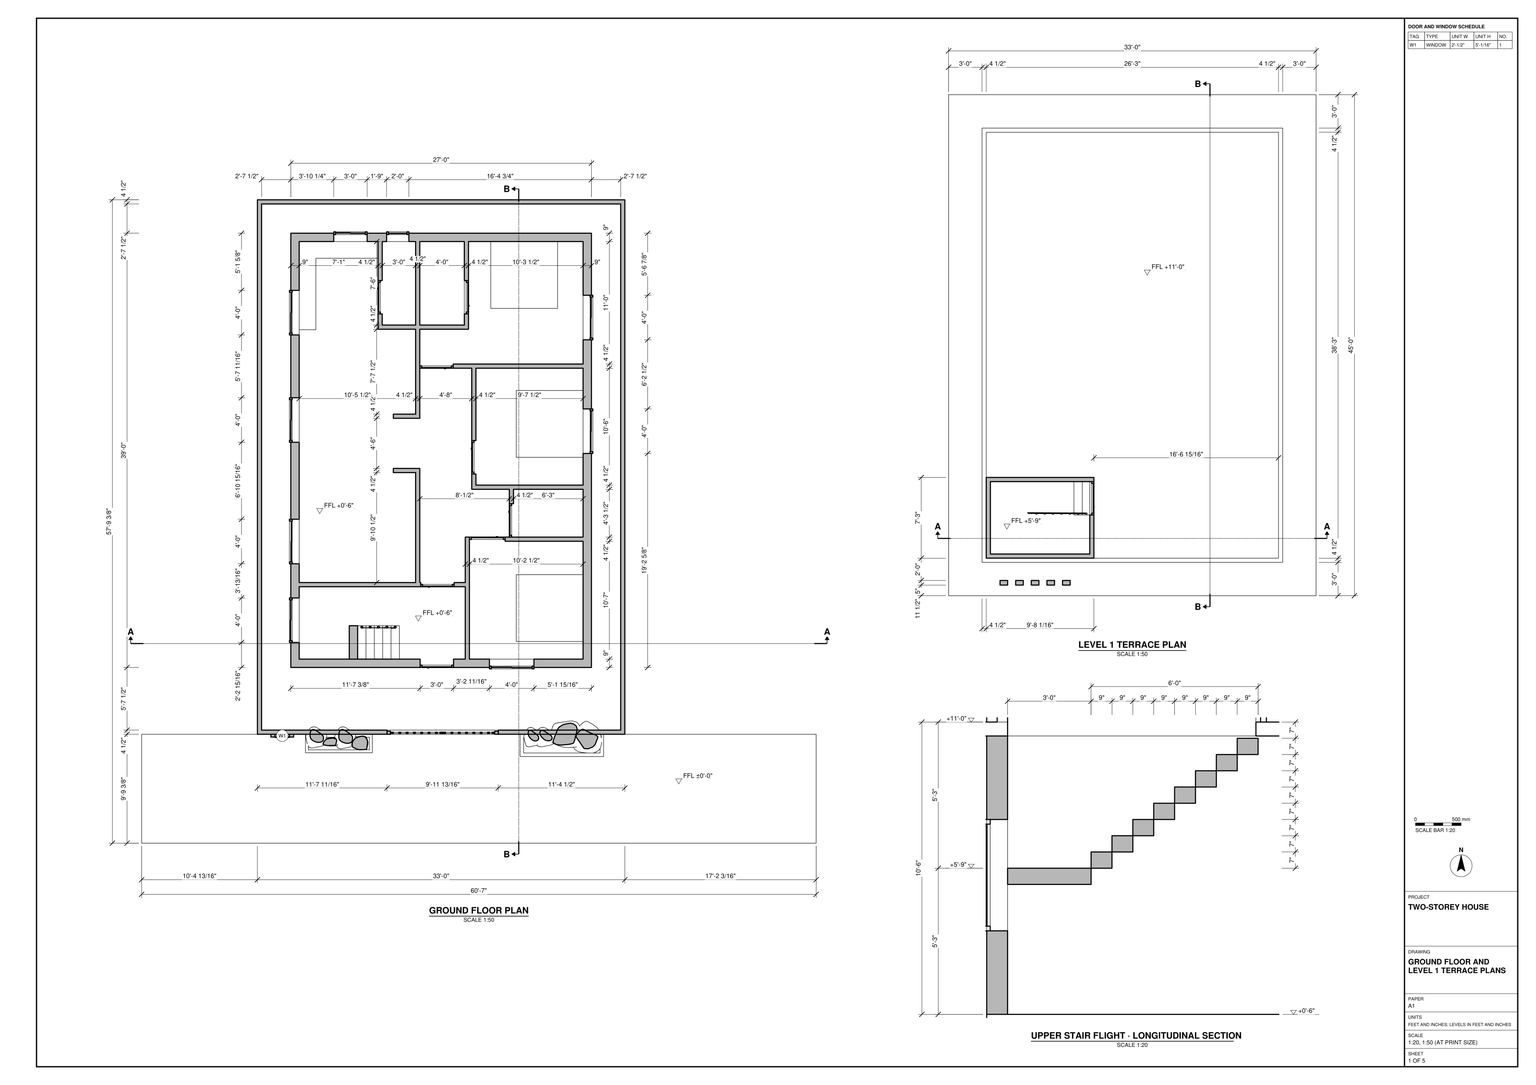
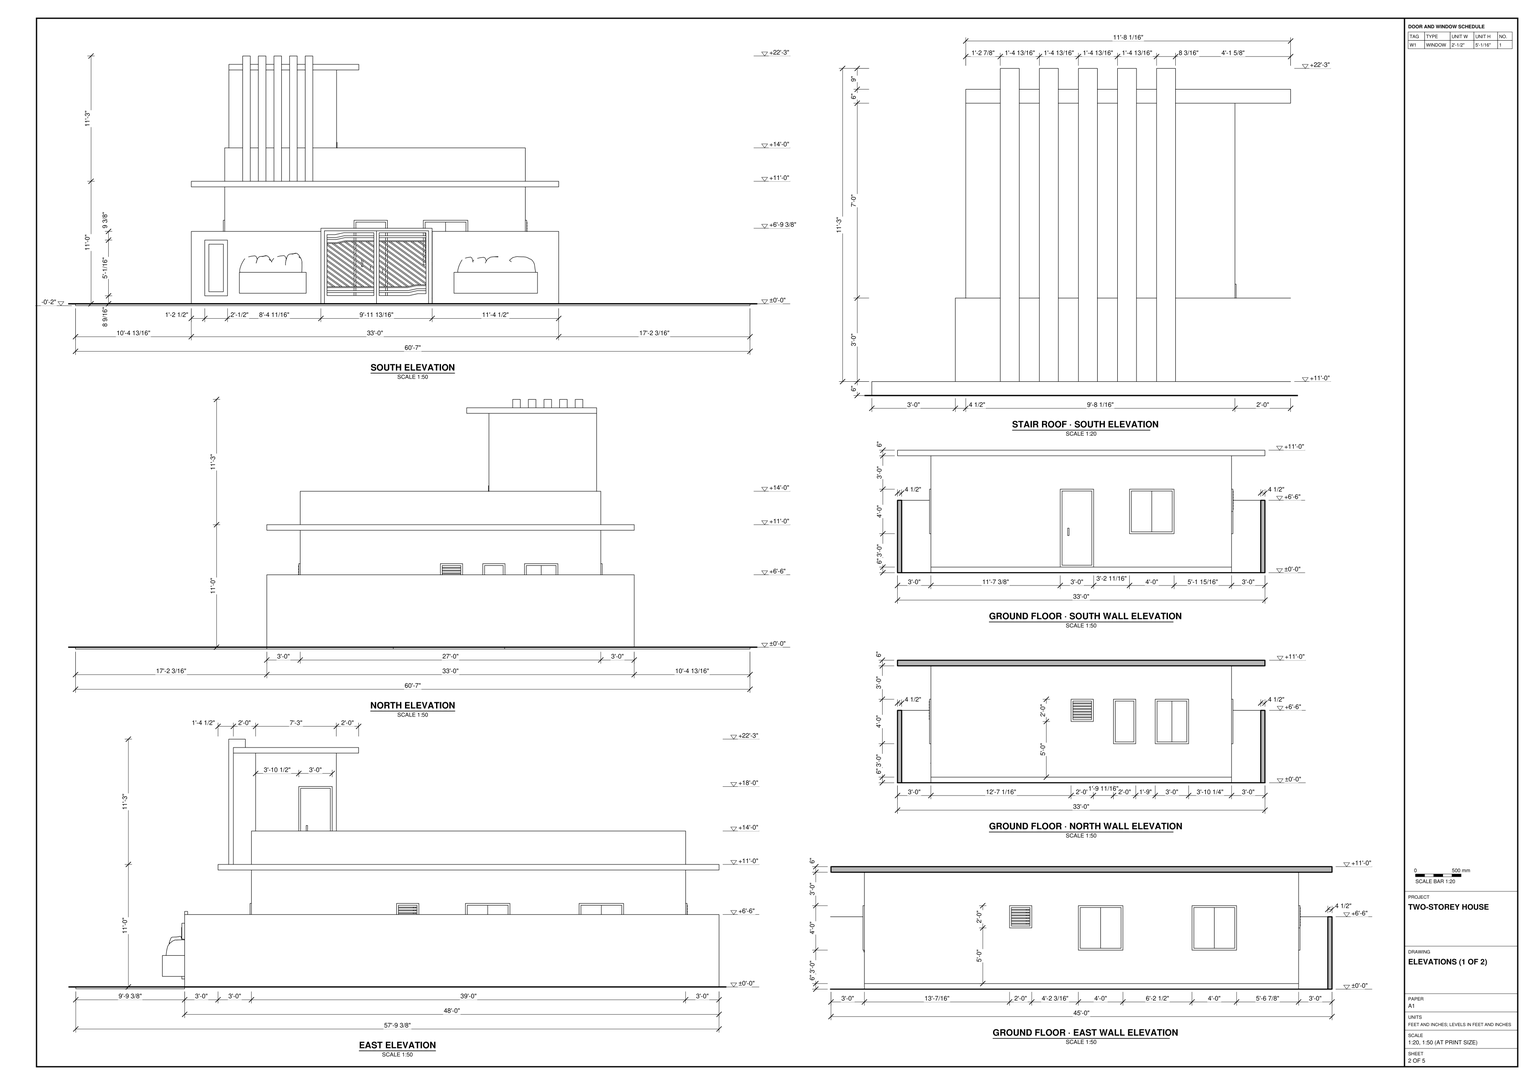
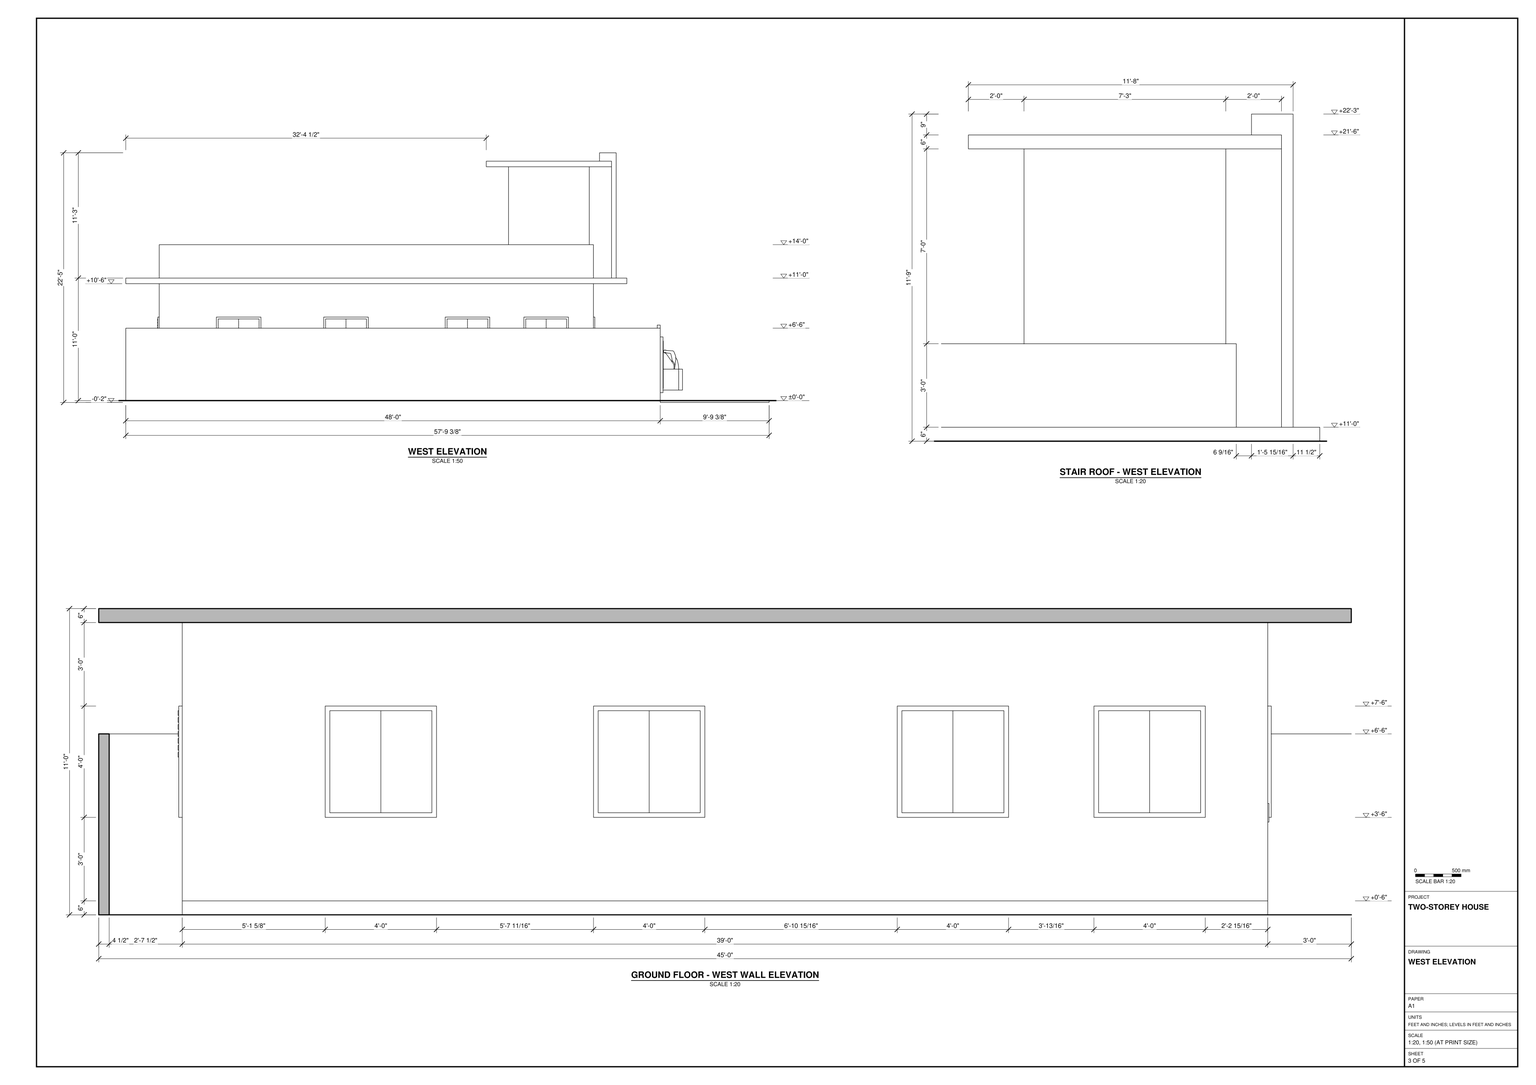
Build the house and its site in SketchUp using task_files/diagram_01.pdf. Work in feet and inches. The overall model, including the ground strip across the front, is 60'-7" wide, 57'-9 3/8" deep and 22'-5" high. Use ±0'-0" as the ground datum and +11'-0" as the terrace level. Set the interior floor at +0'-6", as shown in the ground-floor plan.

Lay out the 27'-0" by 39'-0" house footprint with 9" exterior walls and 4 1/2" interior partitions. Follow the plan for the rooms, connecting passages, built-in joinery and main furniture. Use the individual wall elevations to locate the entrance door, windows and vents. Model the floor slab and the stair near the south entrance, including the intermediate landing at +5'-9". Continue the stair to the enclosure at the southwest corner of the terrace. Show the projecting terrace slab, its inset parapet, and the enclosure’s flat roof and vertical fins.

Model the boundary walls and the double-leaf gate facing south, with a planted box on either side. Decor and loose items, including the plants, may be any suitable library components. Keep shell elements such as walls, slabs and roofs, and each furniture or joinery piece, in separate groups or components. Use components for repeated parts. Save one SketchUp model as output_files/two_storey_house_with_a_roof_terrace_and_gated_frontage.skp.

# SketchUp Ruby script. Lengths in inches.
U = 1.inch
M = Sketchup.active_model
def pt(a) = Geom::Point3d.new(a.map { |v| v * U })
def face(e, loops, mat)
  f = e.add_face(loops[0].map { |a| pt(a) })
  loops[1..].each { |l| e.add_face(l.map { |a| pt(a) }).erase! }
  f.material = f.back_material = mat if mat
  f
end
# faces: each face lists its corners as indices into pts; further lists are holes
def faces(e, pts, list, mat = nil) = list.each { |f| face(e, (f[0].is_a?(Array) ? f : [f]).map { |l| l.map { |i| pts[i] } }, mat) }
# xy, xz, yz: faces in a plane at the given z, y or x. An outline is a flat list of corners, or four numbers for a rectangle; further outlines are holes
def ring(l) = l.size == 4 ? [[l[0], l[1]], [l[2], l[1]], [l[2], l[3]], [l[0], l[3]]] : l.each_slice(2).to_a
def flat(e, list, mat, &to3) = list.each { |f| face(e, (f[0].is_a?(Array) ? f : [f]).map { |l| ring(l).map { |u, v| to3.(u, v) } }, mat) }
def xy(e, z, list, mat = nil) = flat(e, list, mat) { |x, y| [x, y, z] }
def xz(e, y, list, mat = nil) = flat(e, list, mat) { |x, z| [x, y, z] }
def yz(e, x, list, mat = nil) = flat(e, list, mat) { |y, z| [x, y, z] }
def lines(e, pts, list) = list.each { |a, b| e.add_line(pt(pts[a]), pt(pts[b])) }
# prism: a flat outline (further loops are holes) pulled along v
def prism(e, loops, v, mat = nil)
  f = face(e, loops, mat); d = Geom::Vector3d.new(v.map { |x| x * U })
  f.pushpull(f.normal.samedirection?(d) ? d.length : -d.length)
end
def box(e, o, s, mat = nil) = prism(e, [[o, [o[0] + s[0], o[1], o[2]], [o[0] + s[0], o[1] + s[1], o[2]], [o[0], o[1] + s[1], o[2]]]], [0, 0, s[2]], mat)
def at(x, y, z, deg = 0) = Geom::Transformation.translation(pt([x, y, z])) * Geom::Transformation.rotation(ORIGIN, Z_AXIS, deg.degrees)
def axes(o, x, y, z) = Geom::Transformation.new([*x, 0, *y, 0, *z, 0, *pt(o).to_a, 1])
def part(name) = M.definitions.add(name)
# library, detail: a bought-in or finely detailed component or shape, given as its bounding box
def library(name, o, s) = part(name).tap { |d| box(d.entities, o, s) }
def detail(e, o, s) = box(e.add_group.entities, o, s)
def put(e, d, t, mat = nil) = e.add_instance(d, t).tap { |i| i.material = mat if mat }
def group(e, t, mat = nil) = e.add_group.tap { |g| g.transformation = t; g.material = mat if mat }.entities
root = M.entities
M.materials.add("Concrete Simple A01 200cm").color = [121, 120, 120]
M.materials.add("Glass Bronze 001").color = [0, 0, 0]
M.materials["Glass Bronze 001"].alpha = 0.1
M.materials.add("Iron Blurry").color = [53, 53, 53]
M.materials.add("Marble Black 100cm").color = [32, 32, 32]
M.materials.add("Tiles K04 100cm").color = [171, 184, 194]
M.materials.add("Two Color Maple Panels 300cm").color = [56, 46, 41]
M.materials.add("Wall Paint Black Semigloss 300cm").color = [38, 38, 38]
M.materials.add("Wall Paint Bumpy 01 Ochre 100cm").color = [152, 138, 118]
M.materials.add("Wall Paint Dusk Blue Semigloss 300cm").color = [122, 143, 157]
M.materials.add("Wenge Highgloss 300cm").color = [70, 42, 26]
c1 = library("Rubus caesius 001",[-11.39,-9.74,-0.56],[22.57,21.08,20.79])
c2 = library("Scabiosa atropurpurea 005",[-19.05,-18.08,-0.55],[34.7,36.31,33.14])
c3 = library("Skimmia japonica Rubella 004",[-17.08,-16.64,-0.26],[33.2,34.59,28.81])
c4 = library("gate 109k\#1",[0,0.71,0],[103.31,3.23,96.85])
c5 = part("Group\#9")
box(c5.entities,[0,0,0],[0.31,20,2])
c6 = part("Group\#11")
box(c6.entities,[-0.31,0,0],[0.31,22,44])
c7 = part("Group\#13")
box(c7.entities,[-0.31,0,0],[0.31,22,44])
c8 = part("Group\#100")
box(c8.entities,[0,0,0],[20,0.31,2])
c9 = part("Group\#19")
box(c9.entities,[0,-0.31,0],[16,0.31,44])
c10 = part("Group\#21")
box(c10.entities,[0,0,0],[0.31,22,44])
c11 = part("Group\#23")
box(c11.entities,[0,0,0],[0.31,22,44])
c12 = part("Group\#25")
box(c12.entities,[0,0,0],[0.31,22,44])
c13 = part("Group\#27")
box(c13.entities,[0,0,0],[0.31,22,44])
c14 = part("Group\#107")
p = [[63.25,0,0.05],[63.32,0.5,0],[0,0.51,49],[0,0.01,49]]
faces(c14.entities,p,[[0,1,2,3]])
c15 = part("Group\#108")
p = [[63.01,0.5,49],[0,0.82,0],[0,0.32,0],[63.01,0,49]]
faces(c15.entities,p,[[0,1,2,3]])
xy(root,-6,[[124.8125,117.35,264.5,117.35,264.5,121.85,129.3125,121.85,129.3125,688.85,516.3125,688.85,516.3125,121.85,384.5,121.85,384.5,117.35,520.8125,117.35,520.8125,693.35,124.8125,693.35],[264.5,117.35,384.5,121.85]])
xy(root,-6,[[129.3125,121.85,516.3125,688.85]],"Tiles K04 100cm")
xy(root,72,[[124.8125,117.35,264.5,117.35,264.5,121.85,129.3125,121.85,129.3125,688.85,516.3125,688.85,516.3125,121.85,384.5,121.85,384.5,117.35,520.8125,117.35,520.8125,693.35,124.8125,693.35]],"Wall Paint Bumpy 01 Ochre 100cm")
xz(root,117.35,[[124.8125,-6,264.5,72],[384.5,-6,520.8125,72]],"Wall Paint Bumpy 01 Ochre 100cm")
xz(root,121.85,[[129.3125,-6,264.5,72],[384.5,-6,516.3125,72]],"Wall Paint Bumpy 01 Ochre 100cm")
xz(root,688.85,[[129.3125,-6,516.3125,72]],"Wall Paint Bumpy 01 Ochre 100cm")
xz(root,693.35,[[124.8125,-6,520.8125,72]],"Wall Paint Bumpy 01 Ochre 100cm")
yz(root,124.8125,[[117.35,-6,693.35,72]],"Wall Paint Bumpy 01 Ochre 100cm")
yz(root,129.3125,[[121.85,-6,688.85,72]],"Wall Paint Bumpy 01 Ochre 100cm")
yz(root,264.5,[[117.35,-6,121.85,72]],"Wall Paint Bumpy 01 Ochre 100cm")
yz(root,384.5,[[117.35,-6,121.85,72]],"Wall Paint Bumpy 01 Ochre 100cm")
yz(root,516.3125,[[121.85,-6,688.85,72]],"Wall Paint Bumpy 01 Ochre 100cm")
yz(root,520.8125,[[117.35,-6,693.35,72]],"Wall Paint Bumpy 01 Ochre 100cm")
p = [[210.3125,241.85,106],[210.3125,241.53,106]]
lines(root,p,[[0,1]])
put(root,c1,axes([188.29,113.15,19.48],[1,0,0],[0,1.09,0],[0,0,1.29638]))
put(root,c1,axes([219.54,112.67,20.89],[1,0,0],[0,1.13244,0],[0,0,1.23848]))
put(root,c1,axes([421.63,113.52,19.23],[0.85,0,0],[0,1,0],[0,0,1.24]))
put(root,c1,axes([435.05,113.52,19.18],[1,0,0],[0,1,0],[0,0,1.23256]))
put(root,c2,axes([458.75,117.35,13.26],[1,0,0],[0,0.79,0],[0,0,1]))
put(root,c2,axes([236.07,108.0625,24.125],[0.5124,0,0],[0,0.4154,0],[0,0,0.75]))
put(root,c2,axes([204.02,109.2,21.5],[0.5124,0,0],[0,0.25339,0],[0,0,0.75]))
put(root,c3,axes([479.74,113.52,14.77],[1,0,0],[0,1,0],[0,0,1.05505]))
put(root,c4,axes([264.5,116.64,-6],[1.16,0,0],[0,1,0],[0,0,0.84]))
g1 = group(root,at(160.8125,189.35,0))
xy(g1,-2.625,[[139,369,187,459]])
xy(g1,0,[[0,0,0,468,324,468,324,0,175.375,0,175.375,9,188,9,188,87,176,87,176,91.5,188,91.5,188,140.5,192.5,140.5,192.5,9,315,9,315,136,231,136,231,140.5,315,140.5,315,192,240,192,240,176.5,235.5,176.5,235.5,192,195,192,195,208.5,199.5,208.5,199.5,196.5,315,196.5,315,322.5,199.5,322.5,199.5,244.5,195,244.5,195,322.5,175,322.5,175,327,315,327,315,459,191.5,459,191.5,417,187,417,187,459,139,459,139,369,187,369,187,381,191.5,381,191.5,364.5,139,364.5,139,268.5,110.5,268.5,110.5,273,134.5,273,134.5,364.5,94,364.5,94,381,98.5,381,98.5,369,134.5,369,134.5,459,98.5,459,98.5,417,94,417,94,459,9,459,9,91.5,134.5,91.5,134.5,210,110.5,210,110.5,214.5,139,214.5,139,91.5,140,91.5,140,87,9,87,9,9,139.375,9,139.375,0]])
xy(g1,0,[[139.375,0,175.375,0,175.375,9,188,9,188,87,176,87,176,91.5,188,91.5,188,140.5,192.5,140.5,192.5,9,315,9,315,28,243,28,243,100,315,100,315,136,231,136,231,140.5,315,140.5,315,192,240,192,240,176.5,235.5,176.5,235.5,192,195,192,195,208.5,199.5,208.5,199.5,196.5,315,196.5,315,226.5,243,226.5,243,298.5,315,298.5,315,322.5,199.5,322.5,199.5,244.5,195,244.5,195,322.5,175,322.5,175,327,315,327,315,459,287.5,459,287.5,387,215.5,387,215.5,459,191.5,459,191.5,417,187,417,187,381,191.5,381,191.5,364.5,139,364.5,139,268.5,110.5,268.5,110.5,273,134.5,273,134.5,364.5,94,364.5,94,381,98.5,381,98.5,369,134.5,369,134.5,459,98.5,459,98.5,417,94,417,94,459,9,459,9,91.5,134.5,91.5,134.5,210,110.5,210,110.5,214.5,139,214.5,139,91.5,140,91.5,140,87,9,87,9,9,108,9,108,45,117,45,117,9,139.375,9]],"Marble Black 100cm")
xy(g1,36,[[214.0625,0,262.0625,9],[0,26.9375,9,74.9375],[0,111.75,9,159.75],[315,230.625,324,278.625],[0,242.6875,9,290.6875],
  [315,353.125,324,401.125],[0,358.375,9,406.375],[46.25,459,82.25,468],[103.25,459,127.25,468]])
xy(g1,60,[[315,156.4375,324,180.4375],[148.9375,459,172.9375,468]])
xy(g1,84,[[139.375,0,175.375,9],[214.0625,0,262.0625,9],[0,26.9375,9,74.9375],[140,87,176,91.5],[0,111.75,9,159.75],
  [192.5,136,231,140.5],[235.5,140.5,240,176.5],[315,156.4375,324,180.4375],[195,208.5,199.5,244.5],[315,230.625,324,278.625],
  [0,242.6875,9,290.6875],[139,322.5,175,327],[315,353.125,324,401.125],[0,358.375,9,406.375],[94,381,98.5,417],
  [187,381,191.5,417],[46.25,459,82.25,468],[103.25,459,127.25,468],[148.9375,459,172.9375,468]])
xy(g1,120,[[[0,0,324,468],[9,91.5,9,459,94,459,94,364.5,134.5,364.5,134.5,273,110.5,273,110.5,268.5,139,268.5,139,322.5,195,322.5,195,192,235.5,192,235.5,140.5,188,140.5,188,91.5,139,91.5,139,214.5,110.5,214.5,110.5,210,134.5,210,134.5,91.5],[139,327,139,364.5,191.5,364.5,191.5,459,315,459,315,327],[192.5,9,315,136],[199.5,196.5,315,322.5],[9,9,188,87],[139,369,187,459],[240,140.5,315,192],[98.5,369,134.5,459]]])
xz(g1,0,[[[0,0,139.375,0,139.375,84,175.375,84,175.375,0,324,0,324,120,0,120],[214.0625,36,262.0625,84]]],"Wall Paint Dusk Blue Semigloss 300cm")
xz(g1,9,[[9,0,9,120,188,120,188,0,175.375,0,175.375,84,139.375,84,139.375,0],[[192.5,0,315,120],[214.0625,36,262.0625,84]]],"Wall Paint Dusk Blue Semigloss 300cm")
xz(g1,26.9375,[[0,36,9,84]])
xz(g1,74.9375,[[0,36,9,84]])
xz(g1,87,[[9,0,140,0,140,84,176,84,176,0,188,0,188,120,9,120]],"Wall Paint Dusk Blue Semigloss 300cm")
xz(g1,91.5,[[9,0,134.5,120],[139,0,139,120,188,120,188,0,176,0,176,84,140,84,140,0]],"Wall Paint Dusk Blue Semigloss 300cm")
xz(g1,111.75,[[0,36,9,84]])
xz(g1,136,[[231,0,315,0,315,120,192.5,120,192.5,84,231,84]],"Wall Paint Dusk Blue Semigloss 300cm")
xz(g1,140.5,[[188,0,188,120,235.5,120,235.5,84,240,84,240,120,315,120,315,0,231,0,231,84,192.5,84,192.5,0]],"Wall Paint Dusk Blue Semigloss 300cm")
xz(g1,156.4375,[[315,60,324,84]])
xz(g1,159.75,[[0,36,9,84]])
xz(g1,176.5,[[235.5,0,240,84]])
xz(g1,180.4375,[[315,60,324,84]])
xz(g1,192,[[195,0,235.5,120],[240,0,315,120]],"Wall Paint Dusk Blue Semigloss 300cm")
xz(g1,196.5,[[199.5,0,315,120]],"Wall Paint Dusk Blue Semigloss 300cm")
xz(g1,208.5,[[195,0,199.5,84]])
xz(g1,210,[[110.5,0,134.5,120]],"Wall Paint Dusk Blue Semigloss 300cm")
xz(g1,214.5,[[110.5,0,139,120]],"Wall Paint Dusk Blue Semigloss 300cm")
xz(g1,230.625,[[315,36,324,84]])
xz(g1,242.6875,[[0,36,9,84]])
xz(g1,244.5,[[195,0,199.5,84]])
xz(g1,268.5,[[110.5,0,139,120]],"Wall Paint Dusk Blue Semigloss 300cm")
xz(g1,273,[[110.5,0,134.5,120]],"Wall Paint Dusk Blue Semigloss 300cm")
xz(g1,278.625,[[315,36,324,84]])
xz(g1,290.6875,[[0,36,9,84]])
xz(g1,322.5,[[175,0,195,0,195,120,139,120,139,84,175,84],[199.5,0,315,120]],"Wall Paint Dusk Blue Semigloss 300cm")
xz(g1,327,[[175,0,175,84,139,84,139,120,315,120,315,0]],"Wall Paint Dusk Blue Semigloss 300cm")
xz(g1,353.125,[[315,36,324,84]])
xz(g1,358.375,[[0,36,9,84]])
xz(g1,364.5,[[94,0,134.5,120],[139,0,191.5,120]],"Wall Paint Dusk Blue Semigloss 300cm")
xz(g1,369,[[139,-2.625,187,0]])
xz(g1,369,[[98.5,0,134.5,120],[139,0,187,120]],"Wall Paint Dusk Blue Semigloss 300cm")
xz(g1,381,[[94,0,98.5,84],[187,0,191.5,84]])
xz(g1,401.125,[[315,36,324,84]])
xz(g1,406.375,[[0,36,9,84]])
xz(g1,417,[[94,0,98.5,84],[187,0,191.5,84]])
xz(g1,459,[[139,-2.625,187,0]])
xz(g1,459,[[[9,0,94,120],[46.25,36,82.25,84]],[[98.5,0,134.5,120],[103.25,36,127.25,84]],[[139,0,187,120],[148.9375,60,172.9375,84]],[191.5,0,315,120]],"Wall Paint Dusk Blue Semigloss 300cm")
xz(g1,468,[[[0,0,324,120],[46.25,36,82.25,84],[103.25,36,127.25,84],[148.9375,60,172.9375,84]]],"Wall Paint Dusk Blue Semigloss 300cm")
yz(g1,0,[[[0,0,468,120],[111.75,36,159.75,84],[358.375,36,406.375,84],[242.6875,36,290.6875,84],[26.9375,36,74.9375,84]]],"Wall Paint Dusk Blue Semigloss 300cm")
yz(g1,9,[[[9,0,87,120],[26.9375,36,74.9375,84]],[[91.5,0,459,120],[111.75,36,159.75,84],[358.375,36,406.375,84],[242.6875,36,290.6875,84]]],"Wall Paint Dusk Blue Semigloss 300cm")
yz(g1,46.25,[[459,36,468,84]])
yz(g1,82.25,[[459,36,468,84]])
yz(g1,94,[[364.5,0,364.5,120,459,120,459,0,417,0,417,84,381,84,381,0]],"Wall Paint Dusk Blue Semigloss 300cm")
yz(g1,98.5,[[369,0,381,0,381,84,417,84,417,0,459,0,459,120,369,120]],"Wall Paint Dusk Blue Semigloss 300cm")
yz(g1,103.25,[[459,36,468,84]])
yz(g1,110.5,[[210,0,214.5,120],[268.5,0,273,120]])
yz(g1,127.25,[[459,36,468,84]])
yz(g1,134.5,[[91.5,0,210,120],[273,0,364.5,120],[369,0,459,120]],"Wall Paint Dusk Blue Semigloss 300cm")
yz(g1,139,[[369,-2.625,459,0]])
yz(g1,139,[[91.5,0,214.5,120],[268.5,0,364.5,0,364.5,120,327,120,327,84,322.5,84,322.5,120,268.5,120],[369,0,459,120]],"Wall Paint Dusk Blue Semigloss 300cm")
yz(g1,139.375,[[0,0,9,84]])
yz(g1,140,[[87,0,91.5,84]])
yz(g1,148.9375,[[459,60,468,84]])
yz(g1,172.9375,[[459,60,468,84]])
yz(g1,175,[[322.5,0,327,84]])
yz(g1,175.375,[[0,0,9,84]])
yz(g1,176,[[87,0,91.5,84]])
yz(g1,187,[[369,-2.625,459,0]])
yz(g1,187,[[369,0,369,120,459,120,459,0,417,0,417,84,381,84,381,0]],"Wall Paint Dusk Blue Semigloss 300cm")
yz(g1,188,[[9,0,87,120],[91.5,0,140.5,120]],"Wall Paint Dusk Blue Semigloss 300cm")
yz(g1,191.5,[[364.5,0,381,0,381,84,417,84,417,0,459,0,459,120,364.5,120]],"Wall Paint Dusk Blue Semigloss 300cm")
yz(g1,192.5,[[9,0,140.5,0,140.5,84,136,84,136,120,9,120]],"Wall Paint Dusk Blue Semigloss 300cm")
yz(g1,195,[[192,0,192,120,322.5,120,322.5,0,244.5,0,244.5,84,208.5,84,208.5,0]],"Wall Paint Dusk Blue Semigloss 300cm")
yz(g1,199.5,[[196.5,0,208.5,0,208.5,84,244.5,84,244.5,0,322.5,0,322.5,120,196.5,120]],"Wall Paint Dusk Blue Semigloss 300cm")
yz(g1,214.0625,[[0,36,9,84]])
yz(g1,231,[[136,0,140.5,84]])
yz(g1,235.5,[[176.5,0,176.5,84,140.5,84,140.5,120,192,120,192,0]],"Wall Paint Dusk Blue Semigloss 300cm")
yz(g1,240,[[176.5,0,192,0,192,120,140.5,120,140.5,84,176.5,84]])
yz(g1,262.0625,[[0,36,9,84]])
yz(g1,315,[[9,0,136,120],[[140.5,0,192,120],[156.4375,60,180.4375,84]],[[196.5,0,322.5,120],[230.625,36,278.625,84]],[[327,0,459,120],[353.125,36,401.125,84]]],"Wall Paint Dusk Blue Semigloss 300cm")
yz(g1,324,[[[0,0,468,120],[230.625,36,278.625,84],[353.125,36,401.125,84],[156.4375,60,180.4375,84]]],"Wall Paint Dusk Blue Semigloss 300cm")
g2 = group(g1,at(215.5,387,0))
box(g2,[0,0,0],[72,72,36])
g3 = group(g1,at(243,226.5,0))
box(g3,[0,0,0],[72,72,36])
g4 = group(g1,at(243,28,0))
box(g4,[0,0,0],[72,72,36])
g5 = group(g1,at(214.0625,0,36))
prism(g5,[[[48,-1.5,0],[48,-1.5,48],[0,-1.5,48],[0,-1.5,0]],[[46,-1.5,2],[2,-1.5,2],[2,-1.5,46],[46,-1.5,46]]],[0,3,0],"Iron Blurry")
g6 = group(g5,at(2,0,2),"Glass Bronze 001")
box(g6,[0,0,0],[22,0.31,44])
g7 = group(g5,at(24,-0.31,2),"Iron Blurry")
box(g7,[0,0,0],[22,0.31,44],"Glass Bronze 001")
g8 = group(g5,at(109.9375,156.4375,24))
prism(g8,[[[1.5,24,24],[1.5,0,24],[1.5,0,0],[1.5,24,0]],[[1.5,22,22],[1.5,22,2],[1.5,2,2],[1.5,2,22]]],[-3,0,0],"Iron Blurry")
put(g8,c5,at(1.5,2,20),"Glass Bronze 001")
put(g8,c5,at(1.5,2,17),"Glass Bronze 001")
put(g8,c5,at(1.5,2,14),"Glass Bronze 001")
put(g8,c5,at(1.5,2,11),"Glass Bronze 001")
put(g8,c5,at(1.5,2,8),"Glass Bronze 001")
put(g8,c5,at(1.5,2,5),"Glass Bronze 001")
put(g8,c5,at(1.5,2,2),"Glass Bronze 001")
g9 = group(g8,at(0,74.1875,-24))
prism(g9,[[[1.5,0,0],[1.5,48,0],[1.5,48,48],[1.5,0,48]],[[1.5,46,46],[1.5,46,2],[1.5,2,2],[1.5,2,46]]],[-3,0,0],"Iron Blurry")
put(g9,c6,at(-0.5,2,2),"Glass Bronze 001")
put(g9,c6,at(-0.19,24,2),"Glass Bronze 001")
g10 = group(g8,at(0,196.6875,-24))
prism(g10,[[[1.5,48,0],[1.5,48,48],[1.5,0,48],[1.5,0,0]],[[1.5,46,46],[1.5,46,2],[1.5,2,2],[1.5,2,46]]],[-3,0,0],"Iron Blurry")
put(g10,c7,at(-0.5,2,2),"Glass Bronze 001")
put(g10,c7,at(-0.19,24,2),"Glass Bronze 001")
g11 = group(g8,at(-175.0625,311.5625,0))
prism(g11,[[[0,1.5,0],[0,1.5,24],[24,1.5,24],[24,1.5,0]],[[22,1.5,2],[22,1.5,22],[2,1.5,22],[2,1.5,2]]],[0,-3,0],"Iron Blurry")
put(g11,c8,at(2,1.5,20),"Glass Bronze 001")
put(g11,c8,at(2,1.5,17),"Glass Bronze 001")
put(g11,c8,at(2,1.5,14),"Glass Bronze 001")
put(g11,c8,at(2,1.5,11),"Glass Bronze 001")
g12 = group(g11,at(2,1.5,8),"Glass Bronze 001")
box(g12,[0,0,0],[20,0.31,2])
put(g11,c8,at(2,1.5,5),"Glass Bronze 001")
put(g11,c8,at(2,1.5,2),"Glass Bronze 001")
g13 = group(g1,at(103.25,468,36))
prism(g13,[[[24,1.5,0],[0,1.5,0],[0,1.5,48],[24,1.5,48]],[[22,1.5,46],[2,1.5,46],[2,1.5,2],[22,1.5,2]]],[0,-3,0],"Iron Blurry")
g14 = group(g13,at(2,0,2),"Glass Bronze 001")
box(g14,[0,-0.31,0],[20,0.31,44])
g15 = group(g1,at(46.25,468,36))
prism(g15,[[[0,1.5,0],[0,1.5,48],[36,1.5,48],[36,1.5,0]],[[2,1.5,46],[2,1.5,2],[34,1.5,2],[34,1.5,46]]],[0,-3,0],"Iron Blurry")
put(g15,c9,at(18,0.125,2),"Glass Bronze 001")
put(g15,c9,at(2,0.44,2),"Glass Bronze 001")
g16 = group(g1,at(0,358.375,36))
prism(g16,[[[-1.5,0,0],[-1.5,0,48],[-1.5,48,48],[-1.5,48,0]],[[-1.5,2,46],[-1.5,2,2],[-1.5,46,2],[-1.5,46,46]]],[3,0,0],"Iron Blurry")
put(g16,c10,at(0.25,24,2),"Glass Bronze 001")
put(g16,c10,at(-0.06,2,2),"Glass Bronze 001")
g17 = group(g1,at(0,242.6875,36))
prism(g17,[[[-1.5,0,0],[-1.5,0,48],[-1.5,48,48],[-1.5,48,0]],[[-1.5,2,46],[-1.5,2,2],[-1.5,46,2],[-1.5,46,46]]],[3,0,0],"Iron Blurry")
put(g17,c11,at(0.0625,24,2),"Glass Bronze 001")
put(g17,c11,at(-0.25,2,2),"Glass Bronze 001")
g18 = group(g1,at(0,111.75,36))
prism(g18,[[[-1.5,48,0],[-1.5,0,0],[-1.5,0,48],[-1.5,48,48]],[[-1.5,46,2],[-1.5,46,46],[-1.5,2,46],[-1.5,2,2]]],[3,0,0],"Iron Blurry")
put(g18,c12,at(0.5,24,2),"Glass Bronze 001")
put(g18,c12,at(0.19,2,2),"Glass Bronze 001")
g19 = group(g1,at(0,26.9375,36))
prism(g19,[[[-1.5,48,0],[-1.5,0,0],[-1.5,0,48],[-1.5,48,48]],[[-1.5,46,2],[-1.5,46,46],[-1.5,2,46],[-1.5,2,2]]],[3,0,0],"Iron Blurry")
put(g19,c13,at(-0.1875,24,2),"Glass Bronze 001")
put(g19,c13,at(-0.5,2,2),"Glass Bronze 001")
g20 = group(g1,at(139.375,0,0))
prism(g20,[[[36,0,0],[36,0,84],[0,0,84],[0,0,0]],[[34,0,82],[34,0,2],[2,0,2],[2,0,82]]],[0,2.5,0],"Iron Blurry")
g21 = group(g20,at(2,0,2))
box(g21,[0,0,0],[32,0.71,80],"Two Color Maple Panels 300cm")
g22 = group(g21,at(6,0,32),"Iron Blurry")
box(g22,[0,-0.5,0],[1.5,0.5,8])
g23 = group(g1,at(140,87,0))
prism(g23,[[[36,0,0],[36,0,84],[0,0,84],[0,0,0]],[[34,0,82],[34,0,2],[2,0,2],[2,0,82]]],[0,2.5,0],"Iron Blurry")
g24 = group(g23,at(2,0,2))
box(g24,[0,0,0],[32,0.71,80],"Two Color Maple Panels 300cm")
g25 = group(g24,at(6,0,32),"Iron Blurry")
box(g25,[0,-0.5,0],[1.5,0.5,8])
g26 = group(g1,at(94,381,0))
prism(g26,[[[0,0,0],[0,0,84],[0,36,84],[0,36,0]],[[0,2,82],[0,2,2],[0,34,2],[0,34,82]]],[2.5,0,0],"Iron Blurry")
g27 = group(g26,at(0,2,2),"Two Color Maple Panels 300cm")
xy(g27,0,[[0,0,0.71,32]])
xy(g27,80,[[0,0,0.71,32]])
xz(g27,0,[[0,0,0.71,80]])
xz(g27,32,[[0,0,0.71,80]])
yz(g27,0,[[0,0,32,80]],"Two Color Maple Panels 300cm")
yz(g27,0.71,[[0,0,32,80]])
g28 = group(g27,at(0,26,32),"Iron Blurry")
box(g28,[-0.5,-1.5,0],[0.5,1.5,8])
g29 = group(g1,at(195,208.5,0))
prism(g29,[[[0,36,0],[0,0,0],[0,0,84],[0,36,84]],[[0,34,82],[0,2,82],[0,2,2],[0,34,2]]],[2.5,0,0],"Iron Blurry")
g30 = group(g29,at(0,2,2))
box(g30,[0,0,0],[0.71,32,80],"Two Color Maple Panels 300cm")
g31 = group(g30,at(0,26,32),"Iron Blurry")
box(g31,[-0.5,-1.5,0],[0.5,1.5,8])
g32 = group(g1,at(192.5,140.5,0))
prism(g32,[[[0,0,0],[0,0,84],[38.5,0,84],[38.5,0,0]],[[2,0,82],[2,0,2],[36.5,0,2],[36.5,0,82]]],[0,-2.5625,0],"Iron Blurry")
g33 = group(g32,at(2,0,2))
box(g33,[0,-0.71,0],[34.5,0.71,80],"Two Color Maple Panels 300cm")
g34 = group(g33,at(28.5,0,32),"Iron Blurry")
box(g34,[-1.5,0,0],[1.5,0.5,8])
g35 = group(g1,at(108,9,0),"Marble Black 100cm")
box(g35,[0,0,0],[9,36,7])
g36 = group(g35,at(3.5,33.5,7),"Wenge Highgloss 300cm")
prism(g36,[[[1.49,0.13,0],[1.25,0.03,0],[0.99,0,0],[0.73,0.04,0],[0.49,0.14,0],[0.29,0.3,0],[0.13,0.51,0],[0.03,0.75,0],[0,1.01,0],[0.04,1.27,0],[0.14,1.51,0],[0.3,1.71,0],[0.51,1.87,0],[0.75,1.97,0],[1.01,2,0],[1.27,1.96,0],[1.51,1.86,0],[1.71,1.7,0],[1.87,1.49,0],[1.97,1.25,0],[2,0.99,0],[1.96,0.73,0],[1.86,0.49,0],[1.7,0.29,0]]],[0,0,36])
g37 = group(g1,at(99,9,7),"Marble Black 100cm")
box(g37,[0,0,0],[9,36,7])
g38 = group(g37,at(3.5,33.5,7),"Wenge Highgloss 300cm")
prism(g38,[[[2,1,0],[1.97,0.74,0],[1.87,0.5,0],[1.71,0.29,0],[1.5,0.13,0],[1.26,0.03,0],[1,0,0],[0.74,0.03,0],[0.5,0.13,0],[0.29,0.29,0],[0.13,0.5,0],[0.03,0.74,0],[0,1,0],[0.03,1.26,0],[0.13,1.5,0],[0.29,1.71,0],[0.5,1.87,0],[0.74,1.97,0],[1,2,0],[1.26,1.97,0],[1.5,1.87,0],[1.71,1.71,0],[1.87,1.5,0],[1.97,1.26,0]]],[0,0,36])
g39 = group(g1,at(90,9,14),"Marble Black 100cm")
box(g39,[0,0,0],[9,36,7])
g40 = group(g39,at(3.5,33.5,7),"Wenge Highgloss 300cm")
prism(g40,[[[0.74,1.97,0],[1,2,0],[1.26,1.97,0],[1.5,1.87,0],[1.71,1.71,0],[1.87,1.5,0],[1.97,1.26,0],[2,1,0],[1.97,0.74,0],[1.87,0.5,0],[1.71,0.29,0],[1.5,0.13,0],[1.26,0.03,0],[1,0,0],[0.74,0.03,0],[0.5,0.13,0],[0.29,0.29,0],[0.13,0.5,0],[0.03,0.74,0],[0,1,0],[0.03,1.26,0],[0.13,1.5,0],[0.29,1.71,0],[0.5,1.87,0]]],[0,0,36])
g41 = group(g1,at(81,9,21),"Marble Black 100cm")
box(g41,[0,0,0],[9,36,7])
g42 = group(g1,at(72,9,28),"Marble Black 100cm")
box(g42,[0,0,0],[9,36,7])
g43 = group(g42,at(3.5,33.5,7),"Wenge Highgloss 300cm")
prism(g43,[[[1.02,0,0],[0.76,0.03,0],[0.52,0.125,0],[0.31,0.28,0],[0.14,0.48,0],[0.04,0.72,0],[0,0.98,0],[0.03,1.24,0],[0.125,1.48,0],[0.28,1.69,0],[0.48,1.86,0],[0.72,1.96,0],[0.98,2,0],[1.24,1.97,0],[1.48,1.875,0],[1.69,1.72,0],[1.86,1.52,0],[1.96,1.28,0],[2,1.02,0],[1.97,0.76,0],[1.875,0.52,0],[1.72,0.31,0],[1.52,0.14,0],[1.28,0.04,0]]],[0,0,36])
g44 = group(g1,at(63,9,35),"Marble Black 100cm")
box(g44,[0,0,0],[9,36,7])
g45 = group(g44,at(3.5,33.5,7))
xy(g45,0,[[1,0,0.74,0.03,0.5,0.13,0.29,0.29,0.13,0.5,0.03,0.74,0,1,0.03,1.26,0.13,1.5,0.29,1.71,0.5,1.87,0.74,1.97,1,2,1.26,1.97,1.5,1.87,1.71,1.71,1.87,1.5,1.97,1.26,2,1,1.97,0.74,1.87,0.5,1.71,0.29,1.5,0.13,1.26,0.03]])
xy(g45,36,[[1,0,1.26,0.03,1.5,0.13,1.71,0.29,1.87,0.5,1.97,0.74,2,1,1.97,1.26,1.87,1.5,1.71,1.71,1.5,1.87,1.26,1.97,1,2,0.74,1.97,0.5,1.87,0.29,1.71,0.13,1.5,0.03,1.26,0,1,0.03,0.74,0.13,0.5,0.29,0.29,0.5,0.13,0.74,0.03]])
p = [[0.5,0.13,0],[0.74,0.03,0],[0.74,0.03,36],[0.5,0.13,36],[1,0,0],[1,0,36],
  [1.26,0.03,0],[1.26,0.03,36],[1.5,0.13,0],[1.5,0.13,36],[0.29,0.29,0],[0.29,0.29,36],
  [1.71,0.29,0],[1.71,0.29,36],[0.13,0.5,0],[0.13,0.5,36],[1.87,0.5,0],[1.87,0.5,36],
  [0.03,0.74,0],[0.03,0.74,36],[1.97,0.74,0],[1.97,0.74,36],[0,1,0],[0,1,36],
  [2,1,0],[2,1,36],[0.03,1.26,0],[0.03,1.26,36],[1.97,1.26,0],[1.97,1.26,36],
  [0.13,1.5,0],[0.13,1.5,36],[1.87,1.5,0],[1.87,1.5,36],[0.29,1.71,0],[0.29,1.71,36],
  [1.71,1.71,0],[1.71,1.71,36],[0.5,1.87,0],[0.5,1.87,36],[1.5,1.87,0],[1.5,1.87,36],
  [0.74,1.97,0],[0.74,1.97,36],[1.26,1.97,0],[1.26,1.97,36],[1,2,0],[1,2,36]]
faces(g45,p,[[0,1,2,3],[1,4,5,2],[4,6,7,5],[6,8,9,7],[10,0,3,11],[8,12,13,9],[14,10,11,15],[12,16,17,13],
  [18,14,15,19],[16,20,21,17],[22,18,19,23],[20,24,25,21],[26,22,23,27],[24,28,29,25],[30,26,27,31],[28,32,33,29],
  [34,30,31,35],[32,36,37,33],[38,34,35,39],[36,40,41,37],[42,38,39,43],[40,44,45,41],[46,42,43,47],[44,46,47,45]],"Wenge Highgloss 300cm")
g46 = group(g1,at(54,9,42),"Marble Black 100cm")
box(g46,[0,0,0],[9,36,7])
g47 = group(g46,at(3.5,33.5,7),"Wenge Highgloss 300cm")
prism(g47,[[[0.66,0.06,0],[0.43,0.18,0],[0.23,0.35,0],[0.09,0.57,0],[0.01,0.82,0],[0,1.08,0],[0.06,1.34,0],[0.18,1.57,0],[0.35,1.76,0],[0.57,1.9,0],[0.82,1.98,0],[1.08,1.99,0],[1.34,1.9375,0],[1.57,1.82,0],[1.76,1.64,0],[1.9,1.42,0],[1.98,1.17,0],[1.99,0.91,0],[1.9375,0.66,0],[1.82,0.43,0],[1.64,0.23,0],[1.42,0.09,0],[1.17,0.01,0],[0.91,0,0]]],[0,0,36])
g48 = group(g1,at(45,9,49),"Marble Black 100cm")
box(g48,[0,0,0],[9,36,7])
g49 = group(g48,at(3.5,33.5,7),"Wenge Highgloss 300cm")
prism(g49,[[[0.03,1.26,0],[0.13,1.5,0],[0.29,1.71,0],[0.5,1.87,0],[0.74,1.97,0],[1,2,0],[1.26,1.97,0],[1.5,1.87,0],[1.71,1.71,0],[1.87,1.5,0],[1.97,1.26,0],[2,1,0],[1.97,0.74,0],[1.87,0.5,0],[1.71,0.29,0],[1.5,0.13,0],[1.26,0.03,0],[1,0,0],[0.74,0.03,0],[0.5,0.13,0],[0.29,0.29,0],[0.13,0.5,0],[0.03,0.74,0],[0,1,0]]],[0,0,36])
g50 = group(g1,at(36,9,56),"Marble Black 100cm")
box(g50,[-27,0,0],[36,78,7])
g51 = group(g1,at(45,51,63),"Marble Black 100cm")
box(g51,[0,0,0],[9,36,7])
g52 = group(g51,at(3.5,0.5,7),"Wenge Highgloss 300cm")
prism(g52,[[[1.94,1.32,0],[2,1.07,0],[1.98,0.81,0],[1.9,0.56,0],[1.75,0.34,0],[1.56,0.17,0],[1.32,0.05,0],[1.07,0,0],[0.81,0.02,0],[0.56,0.1,0],[0.34,0.24,0],[0.17,0.4375,0],[0.05,0.67,0],[0,0.93,0],[0.02,1.1875,0],[0.1,1.4375,0],[0.24,1.65,0],[0.4375,1.83,0],[0.67,1.94,0],[0.93,2,0],[1.1875,1.98,0],[1.4375,1.9,0],[1.65,1.75,0],[1.83,1.56,0]]],[0,0,36])
g53 = group(g1,at(54,51,70),"Marble Black 100cm")
box(g53,[0,0,0],[9,36,7])
g54 = group(g53,at(3.5,0.5,7),"Wenge Highgloss 300cm")
prism(g54,[[[0.52,1.88,0],[0.77,1.97,0],[1.03,2,0],[1.28,1.96,0],[1.52,1.85,0],[1.72,1.6875,0],[1.88,1.48,0],[1.97,1.23,0],[2,0.97,0],[1.96,0.72,0],[1.85,0.48,0],[1.6875,0.27,0],[1.48,0.12,0],[1.23,0.03,0],[0.97,0,0],[0.72,0.04,0],[0.48,0.15,0],[0.27,0.3125,0],[0.12,0.52,0],[0.03,0.77,0],[0,1.03,0],[0.04,1.28,0],[0.15,1.52,0],[0.3125,1.72,0]]],[0,0,36])
g55 = group(g1,at(63,51,77),"Marble Black 100cm")
box(g55,[0,0,0],[9,36,7])
g56 = group(g55,at(3.5,0.5,7),"Wenge Highgloss 300cm")
prism(g56,[[[1.71,1.71,0],[1.87,1.5,0],[1.97,1.26,0],[2,1,0],[1.97,0.74,0],[1.87,0.5,0],[1.71,0.29,0],[1.5,0.13,0],[1.26,0.03,0],[1,0,0],[0.74,0.03,0],[0.5,0.13,0],[0.29,0.29,0],[0.13,0.5,0],[0.03,0.74,0],[0,1,0],[0.03,1.26,0],[0.13,1.5,0],[0.29,1.71,0],[0.5,1.87,0],[0.74,1.97,0],[1,2,0],[1.26,1.97,0],[1.5,1.87,0]]],[0,0,36])
g57 = group(g1,at(72,51,84),"Marble Black 100cm")
box(g57,[0,0,0],[9,36,7])
g58 = group(g57,at(3.5,0.5,7))
prism(g58,[[[1,0,0],[0.74,0.03,0],[0.5,0.13,0],[0.29,0.29,0],[0.13,0.5,0],[0.03,0.74,0],[0,1,0],[0.03,1.26,0],[0.13,1.5,0],[0.29,1.71,0],[0.5,1.87,0],[0.74,1.97,0],[1,2,0],[1.26,1.97,0],[1.5,1.87,0],[1.71,1.71,0],[1.87,1.5,0],[1.97,1.26,0],[2,1,0],[1.97,0.74,0],[1.87,0.5,0],[1.71,0.29,0],[1.5,0.13,0],[1.26,0.03,0]]],[0,0,36],"Wenge Highgloss 300cm")
g59 = group(g1,at(81,51,91),"Marble Black 100cm")
box(g59,[0,0,0],[9,36,7])
g60 = group(g59,at(3.5,0.5,7),"Wenge Highgloss 300cm")
prism(g60,[[[0.29,1.71,0],[0.5,1.87,0],[0.74,1.97,0],[1,2,0],[1.26,1.97,0],[1.5,1.87,0],[1.71,1.71,0],[1.87,1.5,0],[1.97,1.26,0],[2,1,0],[1.97,0.74,0],[1.87,0.5,0],[1.71,0.29,0],[1.5,0.13,0],[1.26,0.03,0],[1,0,0],[0.74,0.03,0],[0.5,0.13,0],[0.29,0.29,0],[0.13,0.5,0],[0.03,0.74,0],[0,1,0],[0.03,1.26,0],[0.13,1.5,0]]],[0,0,36])
g61 = group(g1,at(90,51,98),"Marble Black 100cm")
box(g61,[0,0,0],[9,36,7])
g62 = group(g61,at(3.51,0.51,7),"Wenge Highgloss 300cm")
prism(g62,[[[0.61,0.07,0],[0.38,0.2,0],[0.2,0.38,0],[0.07,0.61,0],[0,0.86,0],[0,1.12,0],[0.07,1.37,0],[0.2,1.6,0],[0.38,1.78,0],[0.61,1.91,0],[0.86,1.98,0],[1.12,1.98,0],[1.37,1.92,0],[1.6,1.79,0],[1.78,1.6,0],[1.91,1.375,0],[1.98,1.125,0],[1.98,0.86,0],[1.92,0.61,0],[1.79,0.38,0],[1.6,0.2,0],[1.375,0.07,0],[1.125,0,0],[0.86,0,0]]],[0,0,36])
g63 = group(g1,at(99,51,105),"Marble Black 100cm")
box(g63,[0,0,0],[9,36,7])
g64 = group(g63,at(3.5,0.5,7),"Wenge Highgloss 300cm")
prism(g64,[[[0.29,1.71,0],[0.5,1.87,0],[0.74,1.97,0],[1,2,0],[1.26,1.97,0],[1.5,1.87,0],[1.71,1.71,0],[1.87,1.5,0],[1.97,1.26,0],[2,1,0],[1.97,0.74,0],[1.87,0.5,0],[1.71,0.29,0],[1.5,0.13,0],[1.26,0.03,0],[1,0,0],[0.74,0.03,0],[0.5,0.13,0],[0.29,0.29,0],[0.13,0.5,0],[0.03,0.74,0],[0,1,0],[0.03,1.26,0],[0.13,1.5,0]]],[0,0,36])
g65 = group(g1,at(108,51,112))
box(g65,[0,0,0],[9,36,7],"Marble Black 100cm")
g66 = group(g65,at(3.5,0.5,7),"Wenge Highgloss 300cm")
prism(g66,[[[0.13,0.5,0],[0.03,0.74,0],[0,1,0],[0.03,1.26,0],[0.13,1.5,0],[0.29,1.71,0],[0.5,1.87,0],[0.74,1.97,0],[1,2,0],[1.26,1.97,0],[1.5,1.87,0],[1.71,1.71,0],[1.87,1.5,0],[1.97,1.26,0],[2,1,0],[1.97,0.74,0],[1.87,0.5,0],[1.71,0.29,0],[1.5,0.13,0],[1.26,0.03,0],[1,0,0],[0.74,0.03,0],[0.5,0.13,0],[0.29,0.29,0]]],[0,0,36])
g67 = group(g1,at(84.5,42.5,28),"Wenge Highgloss 300cm")
prism(g67,[[[1.03,2,0],[1.29,1.96,0],[1.53,1.85,0],[1.73,1.68,0],[1.88,1.47,0],[1.97,1.22,0],[2,0.96,0],[1.96,0.71,0],[1.85,0.47,0],[1.68,0.27,0],[1.47,0.12,0],[1.22,0.03,0],[0.96,0,0],[0.71,0.04,0],[0.47,0.15,0],[0.27,0.32,0],[0.12,0.53,0],[0.03,0.77,0],[0,1.03,0],[0.04,1.29,0],[0.15,1.53,0],[0.32,1.73,0],[0.53,1.88,0],[0.77,1.97,0]]],[0,0,36])
g68 = group(root,at(169.8125,553.35,0))
xy(g68,0,[[0,0,0,95,85,95,85,77,18,77,18,0]])
xy(g68,36,[[0,0,18,0,18,77,85,77,85,95,0,95]],"Marble Black 100cm")
xz(g68,0,[[0,0,18,36]])
xz(g68,77,[[18,0,85,36]])
xz(g68,95,[[0,0,85,36]])
yz(g68,0,[[0,0,95,36]])
yz(g68,18,[[0,0,77,36]])
yz(g68,85,[[77,0,95,36]])
g69 = group(root,at(352.3125,570.35,0))
prism(g69,[[[0,36,84],[0,0,84],[0,0,0],[0,36,0]],[[0,2,2],[0,2,82],[0,34,82],[0,34,2]]],[-2.5,0,0],"Iron Blurry")
g70 = group(g69,at(0,2,2))
box(g70,[-0.71,0,0],[0.71,32,80],"Two Color Maple Panels 300cm")
g71 = group(g70,at(0,6,32),"Iron Blurry")
box(g71,[0,0,0],[0.5,1.5,8])
g72 = group(root,at(299.8125,511.85,0))
prism(g72,[[[36,0,84],[0,0,84],[0,0,0],[36,0,0]],[[2,0,2],[2,0,82],[34,0,82],[34,0,2]]],[0,2.5,0],"Iron Blurry")
g73 = group(g72,at(2,0,2))
box(g73,[0,0,0],[32,0.71,80],"Two Color Maple Panels 300cm")
g74 = group(g73,at(24.5,0,32),"Iron Blurry")
box(g74,[0,-0.5,0],[1.5,0.5,8])
g75 = group(root,at(396.3125,329.85,0))
prism(g75,[[[0,0,84],[0,36,84],[0,36,0],[0,0,0]],[[0,34,2],[0,34,82],[0,2,82],[0,2,2]]],[2.5,0,0],"Iron Blurry")
g76 = group(g75,at(0,2,2))
box(g76,[0,0,0],[0.71,32,80],"Two Color Maple Panels 300cm")
g77 = group(g76,at(0,26,32),"Iron Blurry")
box(g77,[-0.5,-1.5,0],[0.5,1.5,8])
g78 = group(root,at(160.8125,189.35,-6),"Marble Black 100cm")
box(g78,[0,0,0],[324,468,6],"Marble Black 100cm")
g79 = group(root,at(205.8125,232.98,63))
xy(g79,0,[[0,-0.13,0,7.37,0.31,7.37,0.31,0.18,3.75,0.18,3.75,-0.13]])
xy(g79,7,[[0,7.37,0,9.31,3.6,9.31,3.6,8.99,0.31,8.99,0.31,7.37]])
xy(g79,28.25,[[0,-0.13,3.75,-0.13,3.75,0.18,0.31,0.18,0.31,8.99,3.6,8.99,3.6,9.31,0,9.31]])
xz(g79,-0.13,[[0,0,3.75,28.25]])
xz(g79,0.18,[[0.31,0,3.75,28.25]])
xz(g79,7.37,[[0,0,0.31,7]])
xz(g79,8.99,[[0.31,7,3.6,28.25]])
xz(g79,9.31,[[0,7,3.6,28.25]])
yz(g79,0,[[-0.13,0,-0.13,28.25,9.31,28.25,9.31,7,7.37,7,7.37,0]])
yz(g79,0.31,[[0.18,0,7.37,0,7.37,7,8.99,7,8.99,28.25,0.18,28.25]])
yz(g79,3.6,[[8.99,7,9.31,28.25]])
yz(g79,3.75,[[-0.13,0,0.18,28.25]])
g80 = group(root,at(210.24,232.34,43.72))
p = [[63.25,0,0.05],[63.32,0.5,0],[0,0.51,49],[0,0.01,49]]
faces(g80,p,[[0,1,2,3]])
put(root,c14,at(210.81,231.53,37.8))
put(root,c14,at(210.57,231.875,31.82))
put(root,c14,at(210.57,231.875,25.82))
put(root,c14,at(210.57,231.87,19.82))
put(root,c14,at(210.57,231.87,13.82))
g81 = group(root,at(210.3125,241.53,106))
p = [[63.01,0.5,49],[0,0.82,0],[0,0.32,0],[63.01,0,49]]
faces(g81,p,[[0,1,2,3]])
put(root,c15,at(210.54,241.7,100.01))
put(root,c15,at(209.98,242.03,94.04))
put(root,c15,at(209.98,242.03,88.04))
put(root,c15,at(209.79,242.23,82.05))
put(root,c15,at(209.8,242.22,76.05))
g82 = group(root,at(407.92,117.35,5.33),"Wenge Highgloss 300cm")
xy(g82,0,[[0,-24,90,0]],"Wenge Highgloss 300cm")
xy(g82,5,[[3.83,-20.17,86.17,-3.83]],"Wenge Highgloss 300cm")
xy(g82,22.5625,[[[0,-24,90,0],[3.83,-20.17,86.17,-3.83]]],"Wenge Highgloss 300cm")
xz(g82,-24,[[0,0,90,22.5625]],"Wenge Highgloss 300cm")
xz(g82,-20.17,[[3.83,5,86.17,22.5625]],"Wenge Highgloss 300cm")
xz(g82,-3.83,[[3.83,5,86.17,22.5625]],"Wenge Highgloss 300cm")
xz(g82,0,[[0,0,90,22.5625]],"Wenge Highgloss 300cm")
yz(g82,0,[[-24,0,0,22.5625]],"Wenge Highgloss 300cm")
yz(g82,3.83,[[-20.17,5,-3.83,22.5625]],"Wenge Highgloss 300cm")
yz(g82,86.17,[[-20.17,5,-3.83,22.5625]],"Wenge Highgloss 300cm")
yz(g82,90,[[-24,0,0,22.5625]],"Wenge Highgloss 300cm")
g83 = group(root,at(139.32,117.35,2.55))
xy(g83,0,[[0,-3,24.5,0]],"Iron Blurry")
xy(g83,4.42,[[4.42,-3,20.08,0]],"Iron Blurry")
xy(g83,55.64,[[4.42,-3,20.08,0]],"Iron Blurry")
xy(g83,60.0625,[[0,-3,24.5,0]],"Iron Blurry")
xz(g83,-3,[[[0,0,24.5,60.0625],[4.42,4.42,20.08,55.64]]],"Iron Blurry")
xz(g83,0,[[4.42,4.42,20.08,55.64]])
xz(g83,0,[[[0,0,24.5,60.0625],[4.42,4.42,20.08,55.64]]],"Iron Blurry")
yz(g83,0,[[-3,0,0,60.0625]],"Iron Blurry")
yz(g83,4.42,[[-3,4.42,0,55.64]],"Iron Blurry")
yz(g83,20.08,[[-3,4.42,0,55.64]],"Iron Blurry")
yz(g83,24.5,[[-3,0,0,60.0625]],"Iron Blurry")
g84 = group(root,at(176.61,117.35,5.33),"Wenge Highgloss 300cm")
xy(g84,0,[[0,-19.92,72,0]],"Wenge Highgloss 300cm")
xy(g84,5,[[3.0625,-16.74,68.9375,-3.18]],"Wenge Highgloss 300cm")
xy(g84,22.5625,[[[0,-19.92,72,0],[3.0625,-16.74,68.9375,-3.18]]],"Wenge Highgloss 300cm")
xz(g84,-19.92,[[0,0,72,22.5625]],"Wenge Highgloss 300cm")
xz(g84,-16.74,[[3.0625,5,68.9375,22.5625]],"Wenge Highgloss 300cm")
xz(g84,-3.18,[[3.0625,5,68.9375,22.5625]],"Wenge Highgloss 300cm")
xz(g84,0,[[0,0,72,22.5625]],"Wenge Highgloss 300cm")
yz(g84,0,[[-19.92,0,0,22.5625]],"Wenge Highgloss 300cm")
yz(g84,3.0625,[[-16.74,5,-3.18,22.5625]],"Wenge Highgloss 300cm")
yz(g84,68.9375,[[-16.74,5,-3.18,22.5625]],"Wenge Highgloss 300cm")
yz(g84,72,[[-19.92,0,0,22.5625]],"Wenge Highgloss 300cm")
g85 = group(root,at(124.8125,153.35,120))
g86 = group(g85,at(55.39,16.5,42),"Wenge Highgloss 300cm")
prism(g86,[[[8.1875,0,-36],[8.1875,0,90],[8.1875,12.9375,90],[8.1875,12.9375,99],[8.1875,-5,99],[8.1875,-5,-36]]],[-8.1875,0,0],"Wenge Highgloss 300cm")
g87 = group(g85,at(36,36,0))
xy(g87,0,[[[-36,-36,360,504],[9,9,116.0625,87]]])
xy(g87,6,[[116.0625,51,120.5625,87]])
xy(g87,6,[[[-36,-36,360,504],[4.5,4.5,120.5625,91.5]]],"Tiles K04 100cm")
xy(g87,90,[[116.0625,51,120.5625,87]])
xy(g87,126,[[[4.5,4.5,120.5625,91.5],[9,9,116.0625,87]]])
xz(g87,-36,[[-36,0,360,6]],"Marble Black 100cm")
xz(g87,4.5,[[4.5,6,120.5625,126]],"Wall Paint Bumpy 01 Ochre 100cm")
xz(g87,9,[[9,0,116.0625,126]])
xz(g87,51,[[116.0625,6,120.5625,90]])
xz(g87,87,[[9,0,116.0625,126],[116.0625,6,120.5625,90]])
xz(g87,91.5,[[4.5,6,120.5625,126]],"Wall Paint Bumpy 01 Ochre 100cm")
xz(g87,504,[[-36,0,360,6]],"Marble Black 100cm")
yz(g87,-36,[[-36,0,504,6]],"Marble Black 100cm")
yz(g87,4.5,[[4.5,6,91.5,126]],"Wall Paint Bumpy 01 Ochre 100cm")
yz(g87,9,[[9,0,87,126]])
yz(g87,116.0625,[[9,0,9,126,87,126,87,90,51,90,51,6,87,6,87,0]])
yz(g87,120.5625,[[4.5,6,51,6,51,90,87,90,87,6,91.5,6,91.5,126,4.5,126]],"Wall Paint Bumpy 01 Ochre 100cm")
yz(g87,360,[[-36,0,504,6]],"Marble Black 100cm")
g88 = group(g87,at(0,0,6),"Wall Paint Dusk Blue Semigloss 300cm")
prism(g88,[[[324,0,0],[0,0,0],[0,468,0],[324,468,0]],[[319.5,463.5,0],[4.5,463.5,0],[4.5,4.5,0],[319.5,4.5,0]]],[0,0,36],"Wall Paint Dusk Blue Semigloss 300cm")
g89 = group(g87,at(120.5625,51,6))
prism(g89,[[[0,36,0],[0,36,84],[0,0,84],[0,0,0]],[[0,34,2],[0,2,2],[0,2,82],[0,34,82]]],[-2.5,0,0],"Iron Blurry")
g90 = group(g89,at(0,2,2))
box(g90,[-0.71,0,0],[0.71,32,80],"Two Color Maple Panels 300cm")
g91 = group(g90,at(0,6,32),"Iron Blurry")
box(g91,[0,0,0],[0.5,1.5,8])
g92 = group(g85,at(40.5,40.5,126),"Wall Paint Black Semigloss 300cm")
box(g92,[0,-24,0],[140.0625,135,6],"Wall Paint Black Semigloss 300cm")
g93 = group(g85,at(72.23,16.5,42),"Wenge Highgloss 300cm")
prism(g93,[[[8.1875,0,-36],[8.1875,0,90],[8.1875,12.9375,90],[8.1875,12.9375,99],[8.1875,-5,99],[8.1875,-5,-36]]],[-8.1875,0,0],"Wenge Highgloss 300cm")
g94 = group(g85,at(89.08,16.5,42),"Wenge Highgloss 300cm")
prism(g94,[[[8.1875,0,-36],[8.1875,0,90],[8.1875,12.9375,90],[8.1875,12.9375,99],[8.1875,-5,99],[8.1875,-5,-36]]],[-8.1875,0,0],"Wenge Highgloss 300cm")
g95 = group(g85,at(105.92,16.5,42),"Wenge Highgloss 300cm")
prism(g95,[[[8.1875,0,-36],[8.1875,0,90],[8.1875,12.9375,90],[8.1875,12.9375,99],[8.1875,-5,99],[8.1875,-5,-36]]],[-8.1875,0,0],"Wenge Highgloss 300cm")
g96 = group(g85,at(122.76,16.5,42),"Wenge Highgloss 300cm")
prism(g96,[[[8.1875,0,-36],[8.1875,0,90],[8.1875,12.9375,90],[8.1875,12.9375,99],[8.1875,-5,99],[8.1875,-5,-36]]],[-8.1875,0,0],"Wenge Highgloss 300cm")
g97 = group(root,at(143.74,114.35,6.98),"Glass Bronze 001")
box(g97,[0,-0.31,0],[15.66,0.31,51.22])
g98 = group(root,at(124.8125,0,-6),"Concrete Simple A01 200cm")
prism(g98,[[[-124.8125,117.35,-2],[139.68,117.35,-2],[259.68,117.35,-2],[396,117.35,-2],[602.18,117.35,-2],[602.18,0,-2],[-124.8125,0,-2]]],[0,0,2],"Concrete Simple A01 200cm")
